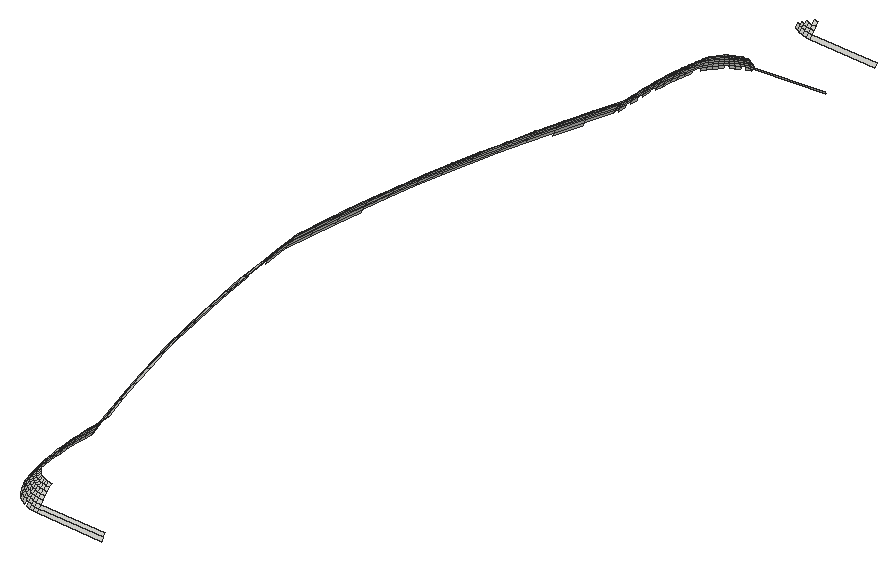
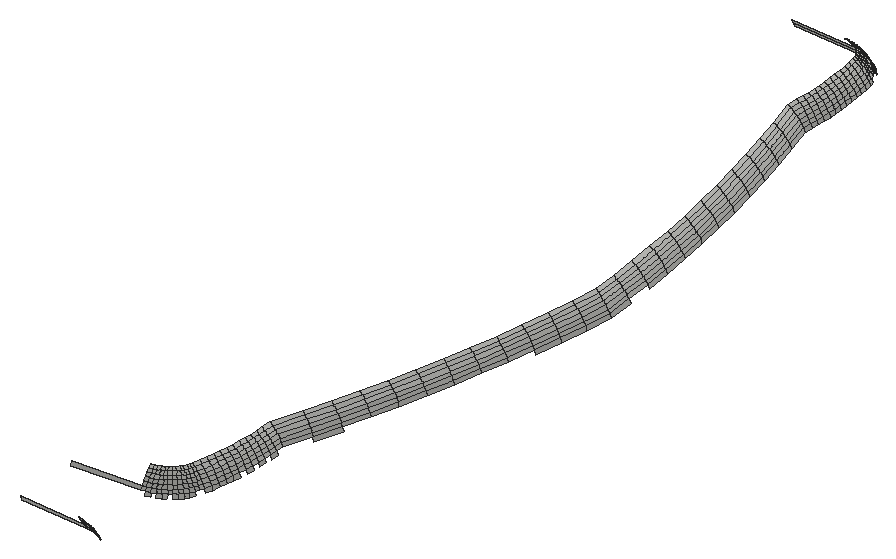
# SketchUp Ruby script. Lengths in inches.
U = 1.inch
M = Sketchup.active_model
def pt(a) = Geom::Point3d.new(a.map { |v| v * U })
def face(e, loops, mat)
  f = e.add_face(loops[0].map { |a| pt(a) })
  loops[1..].each { |l| e.add_face(l.map { |a| pt(a) }).erase! }
  f.material = f.back_material = mat if mat
  f
end
# faces: each face lists its corners as indices into pts; further lists are holes
def faces(e, pts, list, mat = nil) = list.each { |f| face(e, (f[0].is_a?(Array) ? f : [f]).map { |l| l.map { |i| pts[i] } }, mat) }
# xy, xz, yz: faces in a plane at the given z, y or x. An outline is a flat list of corners, or four numbers for a rectangle; further outlines are holes
def ring(l) = l.size == 4 ? [[l[0], l[1]], [l[2], l[1]], [l[2], l[3]], [l[0], l[3]]] : l.each_slice(2).to_a
def flat(e, list, mat, &to3) = list.each { |f| face(e, (f[0].is_a?(Array) ? f : [f]).map { |l| ring(l).map { |u, v| to3.(u, v) } }, mat) }
def xy(e, z, list, mat = nil) = flat(e, list, mat) { |x, y| [x, y, z] }
def xz(e, y, list, mat = nil) = flat(e, list, mat) { |x, z| [x, y, z] }
def yz(e, x, list, mat = nil) = flat(e, list, mat) { |y, z| [x, y, z] }
def lines(e, pts, list) = list.each { |a, b| e.add_line(pt(pts[a]), pt(pts[b])) }
# prism: a flat outline (further loops are holes) pulled along v
def prism(e, loops, v, mat = nil)
  f = face(e, loops, mat); d = Geom::Vector3d.new(v.map { |x| x * U })
  f.pushpull(f.normal.samedirection?(d) ? d.length : -d.length)
end
def box(e, o, s, mat = nil) = prism(e, [[o, [o[0] + s[0], o[1], o[2]], [o[0] + s[0], o[1] + s[1], o[2]], [o[0], o[1] + s[1], o[2]]]], [0, 0, s[2]], mat)
def at(x, y, z, deg = 0) = Geom::Transformation.translation(pt([x, y, z])) * Geom::Transformation.rotation(ORIGIN, Z_AXIS, deg.degrees)
def axes(o, x, y, z) = Geom::Transformation.new([*x, 0, *y, 0, *z, 0, *pt(o).to_a, 1])
def part(name) = M.definitions.add(name)
# library, detail: a bought-in or finely detailed component or shape, given as its bounding box
def library(name, o, s) = part(name).tap { |d| box(d.entities, o, s) }
def detail(e, o, s) = box(e.add_group.entities, o, s)
def put(e, d, t, mat = nil) = e.add_instance(d, t).tap { |i| i.material = mat if mat }
def group(e, t, mat = nil) = e.add_group.tap { |g| g.transformation = t; g.material = mat if mat }.entities
root = M.entities
p = [[331.77,52.04,38.26],[331.77,52,38.17],[330.01,52.11,38.17],[330.01,52.15,38.26],[329.9,52.16,38.26],[329.89,52.12,38.17],
  [329.77,52.15,38.17],[329.79,52.1875,38.26],[329.58,52.28,38.26],[329.56,52.24,38.17],[329.46,52.3,38.17],[329.48,52.34,38.26],
  [329.66,52.19,38.17],[329.68,52.23,38.26],[329.36,52.38,38.17],[329.39,52.41,38.26],[329.28,52.46,38.17],[329.31,52.49,38.26],
  [329.2,52.55,38.17],[329.23,52.57,38.26],[329.07,52.875,38.26],[329.04,52.86,38.17],[329,52.98,38.17],[329.04,52.99,38.26],
  [328.96,53.17,38.17],[329,53.18,38.26],[328.93,53.36,38.17],[328.97,53.37,38.26],[328.9,53.56,38.17],[328.9375,53.5625,38.26],
  [328.87,53.75,38.17],[328.91,53.76,38.26],[328.85,53.95,38.17],[328.89,53.95,38.26],[328.83,54.14,38.17],[328.87,54.15,38.26],
  [328.82,54.34,38.17],[328.86,54.34,38.26],[328.8125,54.53,38.17],[328.85,54.54,38.26],[328.8125,54.73,38.17],[328.85,54.73,38.26],
  [328.8125,54.93,38.17],[328.85,54.93,38.26],[328.82,55.125,38.17],[328.86,55.12,38.26],[328.83,55.34,38.17],[328.875,55.34,38.26],
  [328.61,56.05,38.17],[328.65,56.06,38.26],[328.4,56.74,38.17],[328.44,56.75,38.26],[328.21,57.4375,38.17],[328.25,57.45,38.26],
  [328.03,58.14,38.17],[328.07,58.15,38.26],[327.87,58.84,38.17],[327.91,58.85,38.26],[327.72,59.55,38.17],[327.75,59.5625,38.26],
  [327.58,60.26,38.17],[327.62,60.27,38.26],[327.45,60.98,38.17],[327.49,60.98,38.26],[327.34,61.69,38.17],[327.38,61.7,38.26],
  [327.24,62.41,38.17],[327.28,62.42,38.26],[327.2,63.13,38.26],[327.16,63.13,38.17],[327.09,63.84,38.17],[327.13,63.84,38.26],
  [327.16,64.56,38.17],[327.2,64.55,38.26],[327.24,65.28,38.17],[327.28,65.27,38.26],[327.34,65.99,38.17],[327.38,65.99,38.26],
  [328.44,70.94,38.26],[328.4,70.95,38.17],[328.61,71.64,38.17],[328.65,71.63,38.26],[328.86,72.5625,38.26],[328.82,72.5625,38.17],
  [328.8125,72.76,38.17],[328.85,72.76,38.26],[328.85,72.96,38.26],[328.8125,72.96,38.17],[328.8125,73.15,38.17],[328.85,73.15,38.26],
  [328.86,73.35,38.26],[328.82,73.35,38.17],[328.83,73.54,38.17],[328.87,73.54,38.26],[328.89,73.74,38.26],[328.85,73.74,38.17],
  [328.87,73.93,38.17],[328.91,73.93,38.26],[328.9,74.13,38.17],[328.9375,74.125,38.26],[328.93,74.32,38.17],[328.97,74.32,38.26],
  [328.96,74.52,38.17],[329,74.51,38.26],[329,74.71,38.17],[329.04,74.7,38.26],[329.12,74.92,38.26],[329.08,74.93,38.17],
  [329.13,75.04,38.17],[329.17,75.02,38.26],[329.2,75.14,38.17],[329.23,75.11,38.26],[329.28,75.23,38.17],[329.31,75.2,38.26],
  [329.36,75.31,38.17],[329.39,75.28,38.26],[329.48,75.35,38.26],[329.46,75.38,38.17],[329.56,75.44,38.17],[329.58,75.41,38.26],
  [329.66,75.5,38.17],[329.68,75.46,38.26],[329.79,75.5,38.26],[329.77,75.54,38.17],[329.89,75.5625,38.17],[329.9,75.52,38.26],
  [331.77,77.29,38.26],[331.77,77.25,38.17],[330.01,77.36,38.17],[330.01,77.4,38.26],[329.68,77.48,38.26],[329.66,77.44,38.17],
  [329.56,77.49,38.17],[329.58,77.53,38.26],[329.79,77.4375,38.26],[329.77,77.4,38.17],[329.9,77.41,38.26],[329.89,77.37,38.17],
  [329.46,77.55,38.17],[329.48,77.59,38.26],[331.78,52.09,38.34],[330.02,52.19,38.34],[329.91,52.21,38.34],[329.7,52.27,38.34],
  [329.6,52.32,38.34],[329.8,52.23,38.34],[329.8125,52.28,38.42],[329.72,52.32,38.42],[329.92,52.26,38.42],[330.02,52.25,38.42],
  [329.5,52.375,38.34],[329.42,52.44,38.34],[329.625,52.36,38.42],[329.54,52.42,38.42],[329.34,52.52,38.34],[329.45,52.48,38.42],
  [329.38,52.55,38.42],[329.27,52.6,38.34],[329.3125,52.63,38.42],[329.17,52.67,38.26],[329.21,52.69,38.34],[329.25,52.72,38.42],
  [329.12,52.77,38.26],[329.16,52.79,38.34],[329.21,52.8125,38.42],[329.12,52.89,38.34],[329.17,52.91,38.42],[329.09,53,38.34],
  [329.14,53.01,38.42],[329.05,53.1875,38.34],[329.1,53.2,38.42],[329.01,53.38,38.34],[329.07,53.39,38.42],[328.98,53.57,38.34],
  [329.03,53.58,38.42],[328.96,53.76,38.34],[329.01,53.77,38.42],[328.94,53.95,38.34],[328.99,53.96,38.42],[328.92,54.15,38.34],
  [328.97,54.15,38.42],[328.91,54.34,38.34],[328.96,54.34,38.42],[328.9,54.54,38.34],[328.95,54.54,38.42],[328.9,54.73,38.34],
  [328.95,54.73,38.42],[328.9,54.93,38.34],[328.95,54.92,38.42],[328.91,55.12,38.34],[328.96,55.12,38.42],[328.92,55.35,38.34],
  [328.97,55.35,38.42],[328.69,56.07,38.34],[328.74,56.09,38.42],[328.49,56.76,38.34],[328.54,56.78,38.42],[328.29,57.46,38.34],
  [328.35,57.47,38.42],[328.12,58.16,38.34],[328.17,58.17,38.42],[327.95,58.86,38.34],[328,58.875,38.42],[327.8,59.57,38.34],
  [327.85,59.58,38.42],[327.66,60.28,38.34],[327.71,60.29,38.42],[327.54,60.99,38.34],[327.59,61,38.42],[327.43,61.71,38.34],
  [327.48,61.71,38.42],[327.33,62.42,38.34],[327.38,62.43,38.42],[327.25,63.14,38.34],[327.3,63.14,38.42],[327.18,63.84,38.34],
  [327.23,63.84,38.42],[327.25,64.55,38.34],[327.3,64.54,38.42],[327.33,65.26,38.34],[327.38,65.26,38.42],[327.43,65.98,38.34],
  [327.48,65.97,38.42],[327.54,66.69,38.34],[327.59,66.6875,38.42],[327.49,66.7,38.26],[327.66,67.41,38.34],[327.71,67.4,38.42],
  [327.62,67.41,38.26],[327.75,68.125,38.26],[327.8,68.12,38.34],[327.85,68.11,38.42],[327.95,68.82,38.34],[328,68.8125,38.42],
  [327.91,68.83,38.26],[328.07,69.54,38.26],[328.12,69.53,38.34],[328.17,69.51,38.42],[328.29,70.23,38.34],[328.35,70.21,38.42],
  [328.25,70.24,38.26],[328.49,70.92,38.34],[328.54,70.91,38.42],[328.69,71.62,38.34],[328.74,71.6,38.42],[328.875,72.34,38.26],
  [328.92,72.34,38.34],[328.97,72.33,38.42],[328.91,72.57,38.34],[328.96,72.57,38.42],[328.9,72.76,38.34],[328.95,72.76,38.42],
  [328.9,72.95,38.34],[328.95,72.95,38.42],[328.9,73.15,38.34],[328.95,73.15,38.42],[328.91,73.34,38.34],[328.96,73.34,38.42],
  [328.92,73.54,38.34],[328.97,73.53,38.42],[328.94,73.73,38.34],[328.99,73.73,38.42],[328.96,73.92,38.34],[329.01,73.92,38.42],
  [328.98,74.12,38.34],[329.03,74.11,38.42],[329.01,74.31,38.34],[329.07,74.3,38.42],[329.05,74.5,38.34],[329.1,74.49,38.42],
  [329.09,74.6875,38.34],[329.14,74.67,38.42],[329.07,74.81,38.26],[329.12,74.79,38.34],[329.17,74.78,38.42],[329.16,74.9,38.34],
  [329.21,74.875,38.42],[329.21,74.99,38.34],[329.25,74.97,38.42],[329.27,75.08,38.34],[329.3125,75.05,38.42],[329.34,75.17,38.34],
  [329.38,75.13,38.42],[329.42,75.24,38.34],[329.45,75.2,38.42],[329.5,75.3125,38.34],[329.54,75.27,38.42],[329.6,75.37,38.34],
  [329.625,75.32,38.42],[329.7,75.42,38.34],[329.72,75.37,38.42],[329.8,75.45,38.34],[329.8125,75.4,38.42],[329.91,75.48,38.34],
  [329.92,75.43,38.42],[330.02,75.49,38.34],[330.02,75.44,38.42],[330.01,75.54,38.26],[331.77,75.65,38.26],[331.78,75.6,38.34],
  [329.8,77.48,38.34],[329.7,77.52,38.34],[329.91,77.46,38.34],[330.02,77.44,38.34],[330.02,77.5,38.42],[329.92,77.51,38.42],
  [329.6,77.57,38.34],[329.8125,77.53,38.42],[329.72,77.57,38.42],[330.03,52.3,38.5],[329.93,52.32,38.5],[329.74,52.375,38.5],
  [329.65,52.42,38.5],[329.83,52.34,38.5],[329.57,52.47,38.5],[329.49,52.53,38.5],[329.42,52.59,38.5],[329.36,52.67,38.5],
  [329.31,52.75,38.5],[329.26,52.84,38.5],[329.22,52.93,38.5],[329.2,53.03,38.5],[329.16,53.21,38.5],[329.125,53.4,38.5],
  [329.09,53.59,38.5],[329.07,53.78,38.5],[329.05,53.97,38.5],[329.03,54.16,38.5],[329.02,54.35,38.5],[329.01,54.54,38.5],
  [329.01,54.73,38.5],[329.01,54.92,38.5],[329.02,55.11,38.5],[329.03,55.36,38.5],[328.8,56.1,38.5],[328.59,56.79,38.5],
  [328.4,57.49,38.5],[328.22,58.1875,38.5],[328.06,58.89,38.5],[327.91,59.59,38.5],[327.77,60.3,38.5],[327.65,61.01,38.5],
  [327.54,61.72,38.5],[327.44,62.44,38.5],[327.36,63.15,38.5],[327.29,63.84,38.5],[327.36,64.53,38.5],[327.44,65.25,38.5],
  [327.54,65.96,38.5],[327.65,66.68,38.5],[327.77,67.39,38.5],[327.91,68.09,38.5],[328.06,68.8,38.5],[328.22,69.5,38.5],
  [328.4,70.2,38.5],[328.59,70.89,38.5],[328.8,71.58,38.5],[329.03,72.32,38.5],[329.02,72.57,38.5],[329.01,72.76,38.5],
  [329.01,72.95,38.5],[329.01,73.15,38.5],[329.02,73.34,38.5],[329.03,73.53,38.5],[329.05,73.72,38.5],[329.07,73.91,38.5],
  [329.09,74.1,38.5],[329.125,74.29,38.5],[329.16,74.48,38.5],[329.2,74.66,38.5],[329.22,74.76,38.5],[329.26,74.85,38.5],
  [329.31,74.9375,38.5],[329.36,75.02,38.5],[329.42,75.09,38.5],[329.49,75.16,38.5],[329.57,75.22,38.5],[329.65,75.27,38.5],
  [329.74,75.3125,38.5],[329.83,75.35,38.5],[329.93,75.37,38.5],[330.03,75.38,38.5],[330.03,77.55,38.5],[329.93,77.57,38.5],
  [329.85,52.4,38.57],[329.76,52.43,38.57],[329.9375,52.38,38.57],[330.03,52.37,38.57],[329.68,52.47,38.57],[329.61,52.52,38.57],
  [329.53,52.58,38.57],[329.47,52.64,38.57],[329.41,52.71,38.57],[329.36,52.78,38.57],[329.32,52.86,38.57],[329.29,52.95,38.57],
  [329.26,53.04,38.57],[329.22,53.22,38.57],[329.1875,53.41,38.57],[329.16,53.59,38.57],[329.13,53.78,38.57],[329.11,53.97,38.57],
  [329.09,54.16,38.57],[329.08,54.35,38.57],[329.08,54.54,38.57],[329.07,54.73,38.57],[329.08,54.92,38.57],[329.08,55.11,38.57],
  [329.1,55.37,38.57],[328.86,56.12,38.57],[328.66,56.8125,38.57],[328.47,57.51,38.57],[328.29,58.2,38.57],[328.125,58.9,38.57],
  [327.97,59.61,38.57],[327.84,60.3125,38.57],[327.71,61.02,38.57],[327.6,61.73,38.57],[327.51,62.44,38.57],[327.42,63.16,38.57],
  [327.36,63.84,38.57],[327.42,64.53,38.57],[327.51,65.24,38.57],[327.6,65.96,38.57],[327.71,66.67,38.57],[327.84,67.375,38.57],
  [327.97,68.08,38.57],[328.125,68.78,38.57],[328.29,69.48,38.57],[328.47,70.18,38.57],[328.66,70.875,38.57],[328.86,71.5625,38.57],
  [329.1,72.32,38.57],[329.08,72.58,38.57],[329.08,72.76,38.57],[329.07,72.95,38.57],[329.08,73.14,38.57],[329.08,73.33,38.57],
  [329.09,73.52,38.57],[329.11,73.71,38.57],[329.13,73.9,38.57],[329.16,74.09,38.57],[329.1875,74.28,38.57],[329.22,74.47,38.57],
  [329.26,74.64,38.57],[329.29,74.74,38.57],[329.32,74.82,38.57],[329.36,74.9,38.57],[329.41,74.98,38.57],[329.47,75.05,38.57],
  [329.53,75.11,38.57],[329.61,75.17,38.57],[329.68,75.21,38.57],[329.76,75.25,38.57],[329.85,75.28,38.57],[329.9375,75.3,38.57],
  [330.03,75.32,38.57],[329.79,52.5,38.64],[329.72,52.53,38.64],[329.95,52.45,38.64],[329.87,52.47,38.64],[330.04,52.4375,38.64],
  [330.05,52.51,38.7],[329.96,52.52,38.7],[329.65,52.58,38.64],[329.58,52.63,38.64],[329.75,52.6,38.7],[329.6875,52.64,38.7],
  [329.82,52.57,38.7],[329.89,52.54,38.7],[329.52,52.6875,38.64],[329.47,52.75,38.64],[329.63,52.69,38.7],[329.58,52.74,38.7],
  [329.42,52.82,38.64],[329.53,52.8,38.7],[329.38,52.89,38.64],[329.49,52.86,38.7],[329.45,52.92,38.7],[329.35,52.97,38.64],
  [329.33,53.06,38.64],[329.42,52.99,38.7],[329.29,53.23,38.64],[329.4,53.08,38.7],[329.36,53.25,38.7],[329.26,53.42,38.64],
  [329.33,53.43,38.7],[329.23,53.61,38.64],[329.3,53.62,38.7],[329.2,53.79,38.64],[329.28,53.8,38.7],[329.18,53.98,38.64],
  [329.25,53.99,38.7],[329.16,54.17,38.64],[329.24,54.17,38.7],[329.15,54.35,38.64],[329.23,54.36,38.7],[329.15,54.54,38.64],
  [329.22,54.54,38.7],[329.14,54.73,38.64],[329.22,54.73,38.7],[329.15,54.92,38.64],[329.22,54.92,38.7],[329.15,55.11,38.64],
  [329.23,55.1,38.7],[329.17,55.38,38.64],[329.24,55.39,38.7],[328.93,56.14,38.64],[329,56.16,38.7],[328.72,56.83,38.64],
  [328.8,56.85,38.7],[328.53,57.52,38.64],[328.61,57.54,38.7],[328.36,58.22,38.64],[328.43,58.24,38.7],[328.19,58.92,38.64],
  [328.26,58.93,38.7],[328.04,59.62,38.64],[328.11,59.63,38.7],[327.9,60.32,38.64],[327.98,60.34,38.7],[327.78,61.03,38.64],
  [327.85,61.04,38.7],[327.67,61.74,38.64],[327.75,61.75,38.7],[327.57,62.45,38.64],[327.65,62.46,38.7],[327.49,63.17,38.64],
  [327.57,63.17,38.7],[327.43,63.84,38.64],[327.5,63.84,38.7],[327.49,64.52,38.64],[327.57,64.51,38.7],[327.57,65.23,38.64],
  [327.65,65.22,38.7],[327.67,65.95,38.64],[327.75,65.93,38.7],[327.78,66.65,38.64],[327.85,66.64,38.7],[327.9,67.36,38.64],
  [327.98,67.35,38.7],[328.04,68.07,38.64],[328.11,68.05,38.7],[328.19,68.77,38.64],[328.26,68.75,38.7],[328.36,69.47,38.64],
  [328.43,69.45,38.7],[328.53,70.16,38.64],[328.61,70.14,38.7],[328.72,70.85,38.64],[328.8,70.83,38.7],[328.93,71.54,38.64],
  [329,71.52,38.7],[329.17,72.31,38.64],[329.24,72.3,38.7],[329.15,72.58,38.64],[329.23,72.58,38.7],[329.15,72.77,38.64],
  [329.22,72.77,38.7],[329.14,72.95,38.64],[329.22,72.95,38.7],[329.15,73.14,38.64],[329.22,73.14,38.7],[329.15,73.33,38.64],
  [329.23,73.33,38.7],[329.16,73.52,38.64],[329.24,73.51,38.7],[329.18,73.71,38.64],[329.25,73.7,38.7],[329.2,73.89,38.64],
  [329.28,73.88,38.7],[329.23,74.08,38.64],[329.3,74.07,38.7],[329.26,74.27,38.64],[329.33,74.25,38.7],[329.29,74.45,38.64],
  [329.36,74.4375,38.7],[329.33,74.63,38.64],[329.4,74.61,38.7],[329.35,74.72,38.64],[329.42,74.69,38.7],[329.38,74.79,38.64],
  [329.45,74.76,38.7],[329.42,74.87,38.64],[329.49,74.83,38.7],[329.47,74.9375,38.64],[329.53,74.89,38.7],[329.52,75,38.64],
  [329.58,74.95,38.7],[329.58,75.06,38.64],[329.63,75,38.7],[329.65,75.11,38.64],[329.6875,75.05,38.7],[329.72,75.15,38.64],
  [329.75,75.09,38.7],[329.79,75.1875,38.64],[329.82,75.12,38.7],[329.87,75.22,38.64],[329.89,75.14,38.7],[329.95,75.24,38.64],
  [329.96,75.16,38.7],[330.04,75.25,38.64],[330.05,75.17,38.7]]
faces(root,p,[[0,1,2,3],[4,5,6,7],[3,2,5,4],[8,9,10,11],[7,6,12,13],[11,10,14,15],[15,14,16,17],[17,16,18,19],
  [20,21,22,23],[23,22,24,25],[25,24,26,27],[27,26,28,29],[29,28,30,31],[31,30,32,33],[33,32,34,35],[35,34,36,37],
  [37,36,38,39],[39,38,40,41],[41,40,42,43],[43,42,44,45],[45,44,46,47],[47,46,48,49],[49,48,50,51],[51,50,52,53],
  [53,52,54,55],[55,54,56,57],[57,56,58,59],[59,58,60,61],[61,60,62,63],[63,62,64,65],[65,64,66,67],[68,69,70,71],
  [71,70,72,73],[73,72,74,75],[75,74,76,77],[78,79,80,81],[82,83,84,85],[86,87,88,89],[90,91,92,93],[94,95,96,97],
  [97,96,98,99],[99,98,100,101],[101,100,102,103],[103,102,104,105],[106,107,108,109],[109,108,110,111],[111,110,112,113],[113,112,114,115],
  [116,117,118,119],[119,118,120,121],[122,123,124,125],[126,127,128,129],[130,131,132,133],[134,135,131,130],[136,137,135,134],[129,128,137,136],
  [133,132,138,139],[140,0,3,141],[141,3,4,142],[143,13,8,144],[145,7,13,143],[146,145,143,147],[142,4,7,145],[148,142,145,146],
  [149,141,142,148],[150,11,15,151],[144,8,11,150],[152,144,150,153],[147,143,144,152],[151,15,17,154],[155,151,154,156],[153,150,151,155],
  [154,17,19,157],[156,154,157,158],[157,19,159,160],[158,157,160,161],[160,159,162,163],[161,160,163,164],[163,162,20,165],[164,163,165,166],
  [165,20,23,167],[166,165,167,168],[167,23,25,169],[168,167,169,170],[169,25,27,171],[170,169,171,172],[171,27,29,173],[172,171,173,174],
  [173,29,31,175],[174,173,175,176],[175,31,33,177],[176,175,177,178],[177,33,35,179],[178,177,179,180],[179,35,37,181],[180,179,181,182],
  [181,37,39,183],[182,181,183,184],[183,39,41,185],[184,183,185,186],[186,185,187,188],[185,41,43,187],[188,187,189,190],[187,43,45,189],
  [189,45,47,191],[190,189,191,192],[191,47,49,193],[192,191,193,194],[193,49,51,195],[194,193,195,196],[195,51,53,197],[196,195,197,198],
  [197,53,55,199],[198,197,199,200],[199,55,57,201],[200,199,201,202],[201,57,59,203],[202,201,203,204],[203,59,61,205],[204,203,205,206],
  [205,61,63,207],[206,205,207,208],[207,63,65,209],[208,207,209,210],[209,65,67,211],[210,209,211,212],[211,67,68,213],[212,211,213,214],
  [213,68,71,215],[214,213,215,216],[215,71,73,217],[216,215,217,218],[218,217,219,220],[217,73,75,219],[220,219,221,222],[219,75,77,221],
  [222,221,223,224],[221,77,225,223],[224,223,226,227],[223,225,228,226],[226,228,229,230],[227,226,230,231],[231,230,232,233],[230,229,234,232],
  [232,234,235,236],[233,232,236,237],[237,236,238,239],[236,235,240,238],[238,240,78,241],[239,238,241,242],[241,78,81,243],[242,241,243,244],
  [243,81,245,246],[244,243,246,247],[247,246,248,249],[246,245,82,248],[248,82,85,250],[249,248,250,251],[250,85,86,252],[251,250,252,253],
  [253,252,254,255],[252,86,89,254],[255,254,256,257],[254,89,90,256],[257,256,258,259],[256,90,93,258],[259,258,260,261],[258,93,94,260],
  [261,260,262,263],[260,94,97,262],[262,97,99,264],[263,262,264,265],[264,99,101,266],[265,264,266,267],[267,266,268,269],[266,101,103,268],
  [269,268,270,271],[268,103,105,270],[270,105,272,273],[271,270,273,274],[274,273,275,276],[273,272,106,275],[275,106,109,277],[276,275,277,278],
  [278,277,279,280],[277,109,111,279],[279,111,113,281],[280,279,281,282],[282,281,283,284],[281,113,115,283],[284,283,285,286],[283,115,116,285],
  [286,285,287,288],[285,116,119,287],[288,287,289,290],[287,119,121,289],[290,289,291,292],[289,121,122,291],[292,291,293,294],[294,293,295,296],
  [291,122,125,293],[293,125,297,295],[295,297,298,299],[300,134,130,301],[302,136,134,300],[303,129,136,302],[304,303,302,305],[301,130,133,306],
  [307,300,301,308],[305,302,300,307],[309,149,148,310],[311,147,152,312],[313,146,147,311],[310,148,146,313],[312,152,153,314],[314,153,155,315],
  [315,155,156,316],[316,156,158,317],[317,158,161,318],[318,161,164,319],[319,164,166,320],[320,166,168,321],[321,168,170,322],[322,170,172,323],
  [323,172,174,324],[324,174,176,325],[325,176,178,326],[326,178,180,327],[327,180,182,328],[328,182,184,329],[329,184,186,330],[330,186,188,331],
  [331,188,190,332],[332,190,192,333],[333,192,194,334],[334,194,196,335],[335,196,198,336],[336,198,200,337],[337,200,202,338],[338,202,204,339],
  [339,204,206,340],[340,206,208,341],[341,208,210,342],[342,210,212,343],[343,212,214,344],[344,214,216,345],[345,216,218,346],[346,218,220,347],
  [347,220,222,348],[348,222,224,349],[349,224,227,350],[350,227,231,351],[351,231,233,352],[352,233,237,353],[353,237,239,354],[354,239,242,355],
  [355,242,244,356],[356,244,247,357],[357,247,249,358],[358,249,251,359],[359,251,253,360],[360,253,255,361],[361,255,257,362],[362,257,259,363],
  [363,259,261,364],[364,261,263,365],[365,263,265,366],[366,265,267,367],[367,267,269,368],[368,269,271,369],[369,271,274,370],[370,274,276,371],
  [371,276,278,372],[372,278,280,373],[373,280,282,374],[374,282,284,375],[375,284,286,376],[376,286,288,377],[377,288,290,378],[378,290,292,379],
  [379,292,294,380],[380,294,296,381],[382,304,305,383],[384,313,311,385],[386,310,313,384],[387,309,310,386],[388,312,314,389],[385,311,312,388],
  [390,315,316,391],[389,314,315,390],[391,316,317,392],[392,317,318,393],[394,319,320,395],[393,318,319,394],[395,320,321,396],[396,321,322,397],
  [397,322,323,398],[398,323,324,399],[399,324,325,400],[400,325,326,401],[401,326,327,402],[402,327,328,403],[403,328,329,404],[404,329,330,405],
  [405,330,331,406],[406,331,332,407],[407,332,333,408],[408,333,334,409],[409,334,335,410],[410,335,336,411],[411,336,337,412],[412,337,338,413],
  [413,338,339,414],[414,339,340,415],[415,340,341,416],[416,341,342,417],[417,342,343,418],[418,343,344,419],[419,344,345,420],[420,345,346,421],
  [421,346,347,422],[422,347,348,423],[423,348,349,424],[424,349,350,425],[425,350,351,426],[426,351,352,427],[427,352,353,428],[428,353,354,429],
  [429,354,355,430],[430,355,356,431],[431,356,357,432],[432,357,358,433],[433,358,359,434],[434,359,360,435],[435,360,361,436],[436,361,362,437],
  [437,362,363,438],[438,363,364,439],[439,364,365,440],[440,365,366,441],[441,366,367,442],[442,367,368,443],[443,368,369,444],[444,369,370,445],
  [445,370,371,446],[446,371,372,447],[447,372,373,448],[448,373,374,449],[449,374,375,450],[450,375,376,451],[451,376,377,452],[452,377,378,453],
  [453,378,379,454],[454,379,380,455],[455,380,381,456],[457,385,388,458],[459,386,384,460],[460,384,385,457],[461,387,386,459],[462,461,459,463],
  [464,389,390,465],[458,388,389,464],[466,458,464,467],[468,457,458,466],[469,460,457,468],[463,459,460,469],[470,391,392,471],[465,390,391,470],
  [472,465,470,473],[467,464,465,472],[471,392,393,474],[473,470,471,475],[474,393,394,476],[475,471,474,477],[477,474,476,478],[476,394,395,479],
  [479,395,396,480],[478,476,479,481],[480,396,397,482],[481,479,480,483],[483,480,482,484],[482,397,398,485],[484,482,485,486],[485,398,399,487],
  [486,485,487,488],[487,399,400,489],[488,487,489,490],[489,400,401,491],[490,489,491,492],[491,401,402,493],[492,491,493,494],[493,402,403,495],
  [494,493,495,496],[495,403,404,497],[496,495,497,498],[497,404,405,499],[498,497,499,500],[500,499,501,502],[499,405,406,501],[502,501,503,504],
  [501,406,407,503],[503,407,408,505],[504,503,505,506],[505,408,409,507],[506,505,507,508],[507,409,410,509],[508,507,509,510],[509,410,411,511],
  [510,509,511,512],[511,411,412,513],[512,511,513,514],[513,412,413,515],[514,513,515,516],[515,413,414,517],[516,515,517,518],[517,414,415,519],
  [518,517,519,520],[519,415,416,521],[520,519,521,522],[521,416,417,523],[522,521,523,524],[523,417,418,525],[524,523,525,526],[525,418,419,527],
  [526,525,527,528],[527,419,420,529],[528,527,529,530],[530,529,531,532],[529,420,421,531],[531,421,422,533],[532,531,533,534],[533,422,423,535],
  [534,533,535,536],[535,423,424,537],[536,535,537,538],[538,537,539,540],[537,424,425,539],[540,539,541,542],[539,425,426,541],[542,541,543,544],
  [541,426,427,543],[543,427,428,545],[544,543,545,546],[546,545,547,548],[545,428,429,547],[548,547,549,550],[547,429,430,549],[550,549,551,552],
  [549,430,431,551],[552,551,553,554],[551,431,432,553],[553,432,433,555],[554,553,555,556],[555,433,434,557],[556,555,557,558],[557,434,435,559],
  [558,557,559,560],[560,559,561,562],[559,435,436,561],[562,561,563,564],[561,436,437,563],[563,437,438,565],[564,563,565,566],[565,438,439,567],
  [566,565,567,568],[567,439,440,569],[568,567,569,570],[569,440,441,571],[570,569,571,572],[572,571,573,574],[571,441,442,573],[573,442,443,575],
  [574,573,575,576],[576,575,577,578],[575,443,444,577],[578,577,579,580],[577,444,445,579],[579,445,446,581],[580,579,581,582],[581,446,447,583],
  [582,581,583,584],[584,583,585,586],[583,447,448,585],[585,448,449,587],[586,585,587,588],[588,587,589,590],[587,449,450,589],[590,589,591,592],
  [592,591,593,594],[589,450,451,591],[591,451,452,593],[594,593,595,596],[596,595,597,598],[598,597,599,600],[593,452,453,595],[595,453,454,597],
  [597,454,455,599],[599,455,456,601],[600,599,601,602]])
